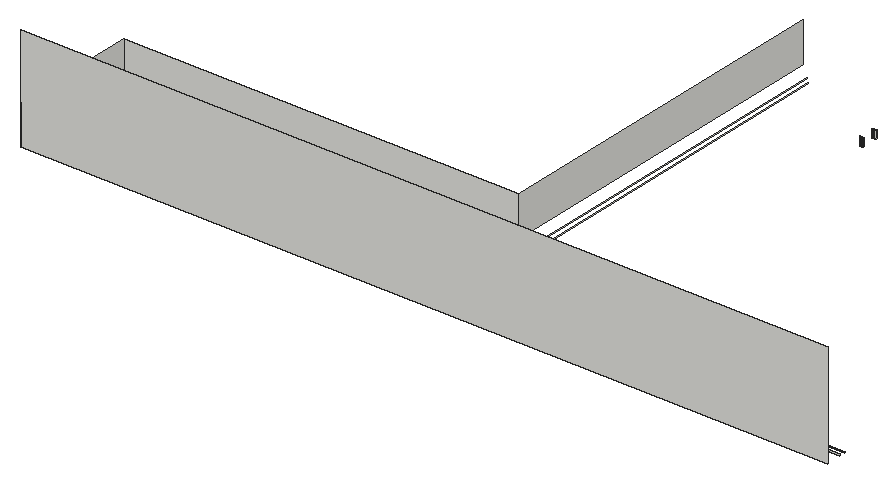
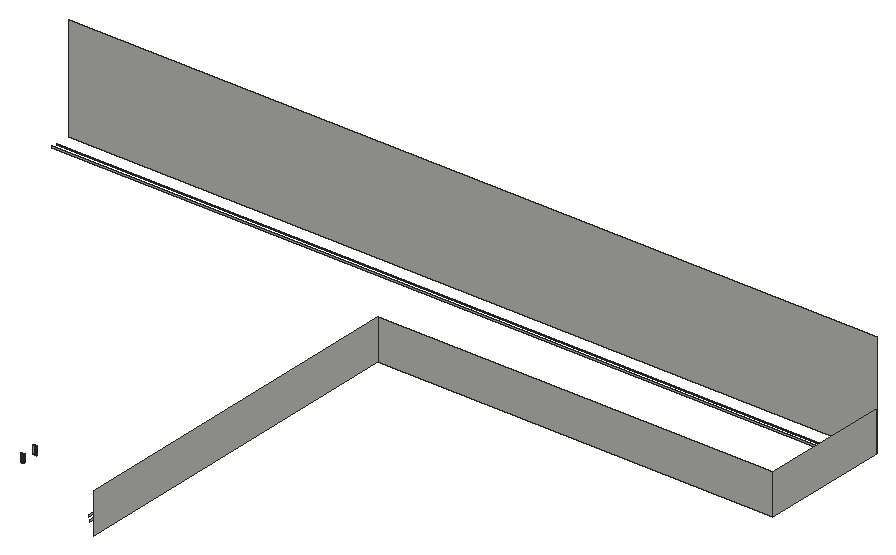
# SketchUp Ruby script. Lengths in inches.
U = 1.inch
M = Sketchup.active_model
def pt(a) = Geom::Point3d.new(a.map { |v| v * U })
def face(e, loops, mat)
  f = e.add_face(loops[0].map { |a| pt(a) })
  loops[1..].each { |l| e.add_face(l.map { |a| pt(a) }).erase! }
  f.material = f.back_material = mat if mat
  f
end
# faces: each face lists its corners as indices into pts; further lists are holes
def faces(e, pts, list, mat = nil) = list.each { |f| face(e, (f[0].is_a?(Array) ? f : [f]).map { |l| l.map { |i| pts[i] } }, mat) }
# xy, xz, yz: faces in a plane at the given z, y or x. An outline is a flat list of corners, or four numbers for a rectangle; further outlines are holes
def ring(l) = l.size == 4 ? [[l[0], l[1]], [l[2], l[1]], [l[2], l[3]], [l[0], l[3]]] : l.each_slice(2).to_a
def flat(e, list, mat, &to3) = list.each { |f| face(e, (f[0].is_a?(Array) ? f : [f]).map { |l| ring(l).map { |u, v| to3.(u, v) } }, mat) }
def xy(e, z, list, mat = nil) = flat(e, list, mat) { |x, y| [x, y, z] }
def xz(e, y, list, mat = nil) = flat(e, list, mat) { |x, z| [x, y, z] }
def yz(e, x, list, mat = nil) = flat(e, list, mat) { |y, z| [x, y, z] }
def lines(e, pts, list) = list.each { |a, b| e.add_line(pt(pts[a]), pt(pts[b])) }
# prism: a flat outline (further loops are holes) pulled along v
def prism(e, loops, v, mat = nil)
  f = face(e, loops, mat); d = Geom::Vector3d.new(v.map { |x| x * U })
  f.pushpull(f.normal.samedirection?(d) ? d.length : -d.length)
end
def box(e, o, s, mat = nil) = prism(e, [[o, [o[0] + s[0], o[1], o[2]], [o[0] + s[0], o[1] + s[1], o[2]], [o[0], o[1] + s[1], o[2]]]], [0, 0, s[2]], mat)
def at(x, y, z, deg = 0) = Geom::Transformation.translation(pt([x, y, z])) * Geom::Transformation.rotation(ORIGIN, Z_AXIS, deg.degrees)
def axes(o, x, y, z) = Geom::Transformation.new([*x, 0, *y, 0, *z, 0, *pt(o).to_a, 1])
def part(name) = M.definitions.add(name)
# library, detail: a bought-in or finely detailed component or shape, given as its bounding box
def library(name, o, s) = part(name).tap { |d| box(d.entities, o, s) }
def detail(e, o, s) = box(e.add_group.entities, o, s)
def put(e, d, t, mat = nil) = e.add_instance(d, t).tap { |i| i.material = mat if mat }
def group(e, t, mat = nil) = e.add_group.tap { |g| g.transformation = t; g.material = mat if mat }.entities
root = M.entities
xz(root,164,[[24,231,324,270]])
xz(root,170,[[30,231,324,231.5]])
xz(root,172,[[32,231,324,231.5]])
xz(root,204,[[32,231,179,231.5]])
xz(root,206,[[30,231,177,231.5]])
xz(root,212,[[24,231,171,246]])
xz(root,317,[[214.28,231,214.35,234],[214.35,231,214.43,234],[214.43,231,214.51,234]])
xz(root,317.01,[[214.12,231,214.2,234],[214.59,231,214.67,234]])
xz(root,322.99,[[214.13,231,214.21,234],[214.6,231,214.68,234]])
xz(root,323,[[214.29,231,214.37,234],[214.37,231,214.45,234],[214.45,231,214.52,234]])
yz(root,24,[[164,231,212,246]])
yz(root,30,[[170,231,206,231.5]])
yz(root,32,[[172,231,204,231.5]])
yz(root,171,[[212,231,344,246]])
yz(root,177,[[206,231,338,231.5]])
yz(root,179,[[204,231,336,231.5]])
p = [[213.89,317.04,231],[213.81,317.06,231],[213.81,317.06,234],[213.89,317.04,234],[213.96,317.03,231],[213.96,317.03,234],
  [214.04,317.02,231],[214.04,317.02,234],[214.12,317.01,231],[214.12,317.01,234],[214.28,317,231],[214.2,317.01,231],
  [214.2,317.01,234],[214.28,317,234],[214.59,317.01,231],[214.51,317,231],[214.51,317,234],[214.59,317.01,234],
  [214.75,317.02,231],[214.67,317.01,231],[214.67,317.01,234],[214.75,317.02,234],[214.82,317.03,231],[214.82,317.03,234],
  [214.9,317.04,231],[214.9,317.04,234],[214.98,317.06,231],[214.98,317.06,234],[213.58,317.11,231],[213.5,317.14,231],
  [213.5,317.14,234],[213.58,317.11,234],[213.66,317.09,231],[213.66,317.09,234],[213.73,317.08,231],[213.73,317.08,234],
  [215.06,317.07,231],[215.06,317.07,234],[215.13,317.09,231],[215.13,317.09,234],[213.52,322.87,231],[213.59,322.89,231],
  [213.59,322.89,234],[213.52,322.87,234],[213.67,322.91,231],[213.67,322.91,234],[213.74,322.93,231],[213.74,322.93,234],
  [213.82,322.94,231],[213.82,322.94,234],[213.9,322.96,231],[213.9,322.96,234],[214.91,322.96,231],[214.99,322.94,231],
  [214.99,322.94,234],[214.91,322.96,234],[215.07,322.92,231],[215.07,322.92,234],[213.98,322.97,231],[213.98,322.97,234],
  [214.05,322.98,231],[214.05,322.98,234],[214.13,322.99,231],[214.13,322.99,234],[214.21,322.99,231],[214.29,323,231],
  [214.29,323,234],[214.21,322.99,234],[214.52,323,231],[214.6,322.99,231],[214.6,322.99,234],[214.52,323,234],
  [214.68,322.99,231],[214.76,322.98,231],[214.76,322.98,234],[214.68,322.99,234],[214.84,322.97,231],[214.84,322.97,234]]
faces(root,p,[[0,1,2,3],[4,0,3,5],[6,4,5,7],[8,6,7,9],[10,11,12,13],[14,15,16,17],[18,19,20,21],[22,18,21,23],
  [24,22,23,25],[26,24,25,27],[28,29,30,31],[32,28,31,33],[34,32,33,35],[1,34,35,2],[36,26,27,37],[38,36,37,39],
  [40,41,42,43],[41,44,45,42],[44,46,47,45],[46,48,49,47],[48,50,51,49],[52,53,54,55],[53,56,57,54],[50,58,59,51],
  [58,60,61,59],[60,62,63,61],[64,65,66,67],[68,69,70,71],[72,73,74,75],[73,76,77,74],[76,52,55,77]])
